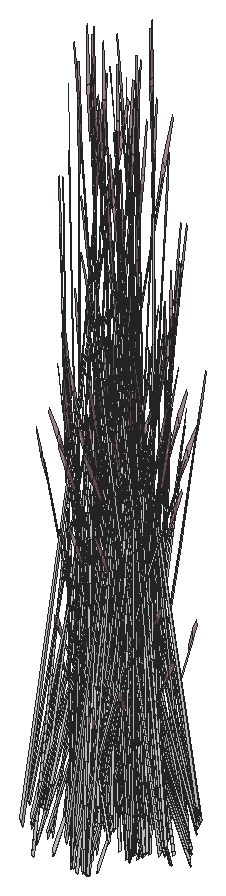
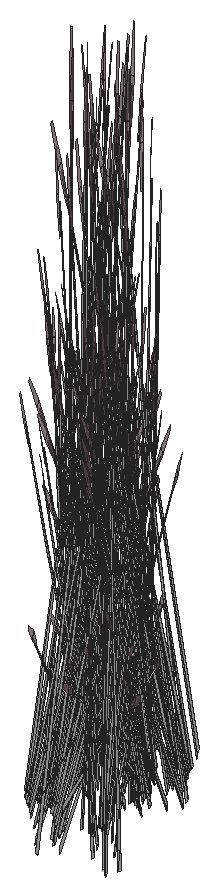
# SketchUp Ruby script. Lengths in inches.
U = 1.inch
M = Sketchup.active_model
def pt(a) = Geom::Point3d.new(a.map { |v| v * U })
def face(e, loops, mat)
  f = e.add_face(loops[0].map { |a| pt(a) })
  loops[1..].each { |l| e.add_face(l.map { |a| pt(a) }).erase! }
  f.material = f.back_material = mat if mat
  f
end
# faces: each face lists its corners as indices into pts; further lists are holes
def faces(e, pts, list, mat = nil) = list.each { |f| face(e, (f[0].is_a?(Array) ? f : [f]).map { |l| l.map { |i| pts[i] } }, mat) }
# xy, xz, yz: faces in a plane at the given z, y or x. An outline is a flat list of corners, or four numbers for a rectangle; further outlines are holes
def ring(l) = l.size == 4 ? [[l[0], l[1]], [l[2], l[1]], [l[2], l[3]], [l[0], l[3]]] : l.each_slice(2).to_a
def flat(e, list, mat, &to3) = list.each { |f| face(e, (f[0].is_a?(Array) ? f : [f]).map { |l| ring(l).map { |u, v| to3.(u, v) } }, mat) }
def xy(e, z, list, mat = nil) = flat(e, list, mat) { |x, y| [x, y, z] }
def xz(e, y, list, mat = nil) = flat(e, list, mat) { |x, z| [x, y, z] }
def yz(e, x, list, mat = nil) = flat(e, list, mat) { |y, z| [x, y, z] }
def lines(e, pts, list) = list.each { |a, b| e.add_line(pt(pts[a]), pt(pts[b])) }
# prism: a flat outline (further loops are holes) pulled along v
def prism(e, loops, v, mat = nil)
  f = face(e, loops, mat); d = Geom::Vector3d.new(v.map { |x| x * U })
  f.pushpull(f.normal.samedirection?(d) ? d.length : -d.length)
end
def box(e, o, s, mat = nil) = prism(e, [[o, [o[0] + s[0], o[1], o[2]], [o[0] + s[0], o[1] + s[1], o[2]], [o[0], o[1] + s[1], o[2]]]], [0, 0, s[2]], mat)
def at(x, y, z, deg = 0) = Geom::Transformation.translation(pt([x, y, z])) * Geom::Transformation.rotation(ORIGIN, Z_AXIS, deg.degrees)
def axes(o, x, y, z) = Geom::Transformation.new([*x, 0, *y, 0, *z, 0, *pt(o).to_a, 1])
def part(name) = M.definitions.add(name)
# library, detail: a bought-in or finely detailed component or shape, given as its bounding box
def library(name, o, s) = part(name).tap { |d| box(d.entities, o, s) }
def detail(e, o, s) = box(e.add_group.entities, o, s)
def put(e, d, t, mat = nil) = e.add_instance(d, t).tap { |i| i.material = mat if mat }
def group(e, t, mat = nil) = e.add_group.tap { |g| g.transformation = t; g.material = mat if mat }.entities
root = M.entities
M.materials.add("LightPink_Translucent").color = [144, 107, 117]
M.materials["LightPink_Translucent"].alpha = 0.75
c1 = part("blade")
p = [[2.15,0.21,22],[0,0.17,0],[0.09,0.45,0],[2.18,0.31,22],[2.29,0.31,22],[0.38,0.45,0],
  [2.48,0.24,33],[2.49,0.24,33],[2.48,0.22,33]]
faces(c1.entities,p,[[0,1,2,3],[4,5,2,3],[6,3,4,7],[8,0,3,6]])
c2 = part("seeds")
p = [[0.3,-0.1,1.38],[-0.01,-0.03,1.59],[-0.01,-0.03,0.03],[0.14,-0.07,-0.07],[0.29,-0.03,3],[0.15,0.01,3.11]]
faces(c2.entities,p,[[0,1,2,3],[1,0,4,5]],"LightPink_Translucent")
c3 = part("blade with seeds")
put(c3.entities,c1,at(0,0,0))
put(c3.entities,c2,axes([2.4,0.25,30.99],[1.5799,-0.05474,1.17369],[-0.12525,1.92788,0.29478],[-0.07173,-0.02425,1.56792]))
put(root,c3,axes([353.46,654.26,621.17],[-0.32928,-0.11539,-0.30978],[0.08291,-0.40636,0.30978],[-0.06638,0.04686,1.38974]))
put(root,c3,axes([350.63,652.3,623.57],[-0.1311,-0.08035,1.71376],[0.27131,-0.33708,0.13857],[0.16909,0.15206,0.73262]))
put(root,c3,axes([349.23,653.36,625.26],[0.21031,-0.39918,-0.1216],[0.30457,0.22997,-0.67495],[0.10587,0.11278,1.02557]))
put(root,c3,axes([355.72,653.76,623.51],[0.10032,-0.06746,1.77064],[0.0346,0.47103,0.13857],[-0.2173,0.0625,0.63284]))
put(root,c3,axes([350.66,651.24,624.16],[-0.30498,-0.24231,1.38283],[0.32203,-0.37727,0.59665],[0.0984,0.22736,1.33663]))
put(root,c3,axes([358.33,656.1875,622.9],[-0.36714,-0.07646,-0.62353],[0.07747,-0.47163,-0.16365],[-0.10956,-0.05715,1.37633]))
put(root,c3,axes([354.74,652.71,621.51],[0.44133,0,0],[0,0.52122,-0.51607],[0,0.11871,1.63711]))
put(root,c3,axes([354.56,652.97,621.34],[-0.44111,-0.00373,-0.04976],[0,-0.52122,0.49943],[-0.01386,0.11865,1.58352]))
put(root,c3,axes([353.61,652.52,621.8],[0.39748,0.22252,-0.29095],[-0.19139,0.46966,-0.50002],[0.01249,0.11531,1.59708]))
put(root,c3,axes([356.57,655.43,622.36],[-0.35581,-0.20937,0],[0.17124,-0.43505,0],[0,0,1.62707]))
put(root,c3,axes([356.86,654.87,622.63],[-0.34464,-0.37536,-0.25192],[0.29,-0.42149,0.5513],[-0.0928,0.04391,1.68216]))
put(root,c3,axes([355.95,655.59,622.65],[0.33032,0.23318,0.49651],[-0.19744,0.41812,0],[-0.07523,-0.05311,1.57504]))
put(root,c3,axes([351.12,653.22,622.46],[-0.19872,-0.13409,1.1486],[0.2566,-0.13625,0.84392],[0.06921,0.11541,0.25299]))
put(root,c3,axes([354.37,653.86,623.66],[0.20082,0.29199,-0.35414],[-0.2293,0.2764,0.4572],[0.1165,0.04206,0.87481]))
put(root,c3,axes([354.47,653.05,621.17],[-0.24637,0.29097,-0.30978],[-0.24637,-0.29097,0.30978],[0,0.09372,1.38974]))
put(root,c3,axes([350.42,653.6,624.73],[0.21031,-0.39918,-0.1216],[0.30457,0.22997,-0.67495],[0.10587,0.11278,1.02557]))
put(root,c3,axes([353.41,653.08,621.8],[0.04113,0.53214,-0.29095],[-0.42835,0.03218,-0.50002],[-0.07543,0.07088,1.59708]))
put(root,c3,axes([354.27,653.97,623.87],[-0.01777,0.35463,0.0643],[-0.26836,-0.00972,0.50621],[0.1028,0.03711,0.77189]))
put(root,c3,axes([357.18,655.31,625.58],[0.09971,-0.42522,0.48003],[0.32782,0.1454,0.3958],[-0.12892,0.02555,0.9933]))
put(root,c3,axes([353.5625,652.87,621.35],[-0.17124,0.42022,-0.44739],[-0.35581,-0.20224,0.21531],[0,0.09687,1.43643]))
put(root,c3,axes([349.98,653.48,621.72],[0.02571,-0.06733,1.76342],[0.32373,-0.19829,-0.26939],[0.09815,0.10263,0.30037]))
put(root,c3,axes([357.15,655.19,625.58],[-0.12963,-0.31798,0.0643],[0.23638,-0.15564,0.50621],[-0.1042,0.03071,0.77189]))
put(root,c3,axes([354.29,653.86,623.87],[-0.26024,0.30729,0.48003],[-0.22444,-0.32634,0.3958],[0.1221,0.05668,0.9933]))
put(root,c3,axes([349.48,653.16,624.91],[0.34827,-0.11086,-0.51099],[0.06092,0.41983,-0.3958],[0.09354,0.12031,0.97773]))
put(root,c3,axes([354.64,654.08,624.88],[-0.05763,0.06055,1.74944],[0.0049,0.44239,-0.27667],[-0.13211,0.05753,0.14031]))
put(root,c3,axes([355.03,654.02,624.85],[-0.09562,0.42421,-0.51099],[-0.32782,-0.1454,-0.3958],[-0.13199,0.0389,0.97773]))
put(root,c3,axes([355.01,653.66,625.2],[0.17758,0.42229,-0.1216],[-0.31518,0.20752,-0.67495],[-0.13282,0.05572,1.02557]))
put(root,c3,axes([357.15,655.52,622.34],[0.00895,0.0735,1.76342],[-0.18044,0.38382,-0.26939],[-0.12817,-0.01935,0.30037]))
put(root,c3,axes([355.76,655.83,622.54],[-0.22066,0.46731,0],[-0.36918,-0.26061,-0.51607],[-0.08408,-0.05936,1.63711]))
put(root,c3,axes([350.15,653.93,624.4],[0.00104,-0.05646,1.77383],[0.30246,-0.2491,-0.16761],[0.10506,0.08891,0.31391]))
put(root,c3,axes([351.18,653.71,621.18],[0.02571,-0.06733,1.76342],[0.32373,-0.19829,-0.26939],[0.09815,0.10263,0.30037]))
put(root,c3,axes([357.9375,656.9,622.875],[-0.08291,-0.40636,-0.30978],[0.32928,-0.11539,0.30978],[-0.06638,-0.04686,1.38974]))
put(root,c3,axes([350.75,652.18,621.79],[0.12941,0.42699,-0.69212],[-0.37279,0.15378,-0.18165],[0.0143,0.14459,1.52773]))
put(root,c3,axes([357.03,654.56,622.89],[0.38326,-0.02879,0.44739],[0.03466,0.47788,-0.21531],[-0.06861,0.04843,1.43643]))
put(root,c3,axes([349.96,653.59,622.89],[-0.22633,-0.01463,1.0506],[0.14947,-0.31064,0.58006],[0.08941,0.11036,0.8241]))
put(root,c3,axes([350.67,653.4,624.37],[0.34827,-0.11086,-0.51099],[0.06092,0.41983,-0.3958],[0.09354,0.12031,0.97773]))
put(root,c3,axes([353.15,653.48,621.2],[-0.23773,0.35053,-0.62353],[-0.29532,-0.31785,-0.16365],[-0.09526,0.08744,1.37633]))
put(root,c3,axes([353.47,654.22,624.1875],[-0.05451,-0.37564,0.35414],[0.31161,-0.09919,-0.4572],[0.0837,0.10765,0.87481]))
put(root,c3,axes([356.6875,654.79,622.38],[-0.38326,0.02879,-0.44739],[-0.03466,-0.47788,0.21531],[-0.06861,0.04843,1.43643]))
put(root,c3,axes([353.57,654.08,621.47],[0.44186,0.15158,0.30756],[-0.11054,0.54181,-0.36492],[-0.07313,0.06781,1.64885]))
put(root,c3,axes([353.54,654.44,621.16],[-0.33032,0.23318,-0.49651],[-0.19744,-0.41812,0],[-0.07523,0.05311,1.57504]))
put(root,c3,axes([354.64,653.0625,621.16],[0,0.46636,-0.49651],[-0.39487,0,0],[0,0.10622,1.57504]))
put(root,c3,axes([353.65,653.11,623.01],[-0.1311,-0.08035,1.71376],[0.27131,-0.33708,0.13857],[0.16909,0.15206,0.73262]))
put(root,c3,axes([357.85,657.08,622.86],[-0.33032,-0.23318,-0.49651],[0.19744,-0.41812,0],[-0.07523,-0.05311,1.57504]))
put(root,c3,axes([357.11,655.35,625.37],[-0.29332,-0.1301,-0.35414],[0.08555,-0.37955,0.4572],[-0.11809,0.0348,0.87481]))
put(root,c3,axes([351.15,653.83,622.36],[-0.22633,-0.01463,1.0506],[0.14947,-0.31064,0.58006],[0.08941,0.11036,0.8241]))
put(root,c3,axes([353.68,652.06,623.61],[-0.30498,-0.24231,1.38283],[0.32203,-0.37727,0.59665],[0.0984,0.22736,1.33663]))
put(root,c3,axes([358.74,656.26,623.51],[-0.35635,0.30962,-0.29095],[-0.23697,-0.43749,-0.50002],[-0.08792,-0.04443,1.59708]))
put(root,c3,axes([350.5,653.74,624.42],[-0.16041,0.29625,0.0643],[-0.22843,-0.17248,0.50621],[0.07385,0.09498,0.77189]))
put(root,c3,axes([354.14,654.03,621.9],[-0.19872,-0.13409,1.1486],[0.2566,-0.13625,0.84392],[0.06921,0.11541,0.25299]))
put(root,c3,axes([353.4375,654.41,624.17],[0.21031,-0.39918,-0.1216],[0.30457,0.22997,-0.67495],[0.10587,0.11278,1.02557]))
put(root,c3,axes([350.57,653.66,624.42],[-0.35104,0.10702,0.48003],[-0.06092,-0.41983,0.3958],[0.08256,0.12373,0.9933]))
put(root,c3,axes([357.11,655.9,622.36],[-0.21791,-0.46895,-0.05142],[0.36918,-0.26061,0.51607],[-0.09097,0.04465,1.6363]))
put(root,c3,axes([357.03,654.77,622.79],[0.26075,0.2802,0.1448],[-0.2175,0.31612,-0.41347],[-0.06054,0.04274,1.26744]))
put(root,c3,axes([354.97,654.84,624.9],[-0.08753,-0.42921,0.48003],[0.34336,-0.07449,0.3958],[-0.1012,0.10094,0.9933]))
put(root,c3,axes([354.91,654.76,624.9],[-0.2423,-0.19613,0.0643],[0.14107,-0.2793,0.50621],[-0.07768,0.0903,0.77189]))
put(root,c3,axes([355.02,654.24,624.04],[0.12246,-0.09864,1.71376],[0.1031,0.45582,0.13857],[-0.19225,0.10302,0.73262]))
put(root,c3,axes([352.05,653.87,624.1875],[0.23881,-0.24554,0.35414],[0.22606,0.28036,-0.4572],[-0.0344,0.14245,0.87481]))
put(root,c3,axes([350.41,653.07,622.28],[0.00623,-0.15459,1.43002],[0.29764,-0.17268,-0.30754],[0.09188,0.18503,0.61141]))
put(root,c3,axes([353.84,654.37,621.51],[0.22066,0.46731,0],[-0.36918,0.26061,-0.51607],[-0.08408,0.05936,1.63711]))
put(root,c3,axes([357.42,655.3125,625.9],[0.29332,0.1301,0.35414],[-0.08555,0.37955,-0.4572],[-0.11809,0.0348,0.87481]))
put(root,c3,axes([353.16,654.74,623.85],[0.00104,-0.05646,1.77383],[0.30246,-0.2491,-0.16761],[0.10506,0.08891,0.31391]))
put(root,c3,axes([354.19,654.53,620.63],[0.02571,-0.06733,1.76342],[0.32373,-0.19829,-0.26939],[0.09815,0.10263,0.30037]))
put(root,c3,axes([353.65,652.52,621.98],[-0.00964,-0.43909,1.41272],[0.43635,0.11382,0.59816],[-0.1032,0.24027,1.3335]))
put(root,c3,axes([353.76,653,621.23],[0.12941,0.42699,-0.69212],[-0.37279,0.15378,-0.18165],[0.0143,0.14459,1.52773]))
put(root,c3,axes([353.6875,654.21,623.82],[0.34827,-0.11086,-0.51099],[0.06092,0.41983,-0.3958],[0.09354,0.12031,0.97773]))
put(root,c3,axes([357.3125,655.63,622.65],[0.33032,-0.23318,0.49651],[0.19744,0.41812,0],[-0.07523,0.05311,1.57504]))
put(root,c3,axes([352.72,654.28,624.1875],[0.1064,-0.35863,0.35414],[0.31043,0.1046,-0.4572],[0.02846,0.14439,0.87481]))
put(root,c3,axes([358,655.29,624.1875],[0.10032,-0.06746,1.77064],[0.0346,0.47103,0.13857],[-0.2173,0.0625,0.63284]))
put(root,c3,axes([357.01,655.84,622.2],[-0.32928,-0.11539,-0.30978],[0.08291,-0.40636,0.30978],[-0.06638,0.04686,1.38974]))
put(root,c3,axes([354.64,655.02,622.76],[0.12266,0.03828,1.43002],[0.07906,0.39104,-0.30754],[-0.16661,0.0732,0.61141]))
put(root,c3,axes([350.82,660.1,620.59],[-0.10032,0.0944,1.43002],[-0.30046,-0.16522,-0.30754],[0.05569,-0.20547,0.61141]))
put(root,c3,axes([355.1875,654.7,625.22],[0.30722,-0.06665,0.35414],[0.08112,0.381,-0.4572],[-0.08804,0.10234,0.87481]))
put(root,c3,axes([354.17,654.64,621.8],[-0.22633,-0.01463,1.0506],[0.14947,-0.31064,0.58006],[0.08941,0.11036,0.8241]))
put(root,c3,axes([354,654.53,624.88],[0.04504,0.01251,1.77383],[0.13934,0.41205,-0.16761],[-0.0922,0.10815,0.31391]))
put(root,c3,axes([355.53,660.61,621.875],[0.08068,0.14973,1.71376],[-0.3728,0.12606,0.13857],[-0.08426,-0.23506,0.73262]))
put(root,c3,axes([357.66,660.63,621.875],[0.08068,0.14973,1.71376],[-0.3728,0.12606,0.13857],[-0.08426,-0.23506,0.73262]))
put(root,c3,axes([353.52,654.56,623.87],[-0.16041,0.29625,0.0643],[-0.22843,-0.17248,0.50621],[0.07385,0.09498,0.77189]))
put(root,c3,axes([354.38,655.84,622.93],[0.14709,-0.21136,1.1486],[0.05804,0.3346,0.84392],[-0.1063,0.05991,0.25299]))
put(root,c3,axes([356.15,659.62,622.72],[-0.05398,-0.06539,1.74944],[-0.36026,0.04145,-0.27667],[-0.0575,-0.15639,0.14031]))
put(root,c3,axes([356.96,654.66,622.83],[0.04113,0.53214,-0.29095],[-0.42835,0.03218,-0.50002],[-0.07543,0.07088,1.59708]))
put(root,c3,axes([353.14,655.55,624.78],[0.2439,-0.26754,-0.06488],[0.22348,0.29302,-0.29416],[0.01573,0.08303,0.97024]))
put(root,c3,axes([357.11,654.45,622.38],[-0.17124,0.42022,-0.44739],[-0.35581,-0.20224,0.21531],[0,0.09687,1.43643]))
put(root,c3,axes([350.09,652.77,623.57],[-0.08068,-0.14973,1.71376],[0.3728,-0.12606,0.13857],[0.08426,0.23506,0.73262]))
put(root,c3,axes([353.58,654.47,623.87],[-0.35104,0.10702,0.48003],[-0.06092,-0.41983,0.3958],[0.08256,0.12373,0.9933]))
put(root,c3,axes([354.93,654.92,624.7],[-0.30722,0.06665,-0.35414],[-0.08112,-0.381,0.4572],[-0.08804,0.10234,0.87481]))
put(root,c3,axes([356.53,660.73,622.98],[-0.16845,-0.3792,-0.71045],[0.34676,-0.21133,0.08574],[-0.03939,-0.18322,1.00501]))
put(root,c3,axes([356.93,655.61,625.56],[-0.05763,0.06055,1.74944],[0.0049,0.44239,-0.27667],[-0.13211,0.05753,0.14031]))
put(root,c3,axes([357.3125,655.55,625.53],[-0.09562,0.42421,-0.51099],[-0.32782,-0.1454,-0.3958],[-0.13199,0.0389,0.97773]))
put(root,c3,axes([357.3,655.18,625.88],[0.17758,0.42229,-0.1216],[-0.31518,0.20752,-0.67495],[-0.13282,0.05572,1.02557]))
put(root,c3,axes([351.06,660.8,622.98],[0.00918,-0.43138,-0.71045],[0.38672,0.02897,0.08574],[0.04081,-0.18275,1.00501]))
put(root,c3,axes([355.43,660.22,620.59],[-0.02137,0.15256,1.43002],[-0.31245,0.12771,-0.30754],[-0.07303,-0.19719,0.61141]))
put(root,c3,axes([358.05,657.36,623.22],[-0.22066,0.46731,0],[-0.36918,-0.26061,-0.51607],[-0.08408,-0.05936,1.63711]))
put(root,c3,axes([357.56,660.23,620.59],[-0.02137,0.15256,1.43002],[-0.31245,0.12771,-0.30754],[-0.07303,-0.19719,0.61141]))
put(root,c3,axes([353.43,653.88,621.73],[0.00623,-0.15459,1.43002],[0.29764,-0.17268,-0.30754],[0.09188,0.18503,0.61141]))
put(root,c3,axes([351.6,660.12,622.72],[-0.00341,-0.09282,1.74944],[-0.28775,-0.26825,-0.27667],[0.04449,-0.16261,0.14031]))
put(root,c3,axes([350.625,660.58,621.875],[-0.06572,0.16029,1.71376],[-0.27569,-0.33172,0.13857],[0.12437,-0.20675,0.73262]))
put(root,c3,axes([351.52,659.79,622.71],[-0.03584,0.03562,1.77383],[-0.35118,-0.12018,-0.16761],[-0.01271,-0.15545,0.31391]))
put(root,c3,axes([356.23,659.88,619.49],[-0.0592,0.0168,1.76342],[-0.32738,-0.18913,-0.26939],[0.00549,-0.15776,0.30037]))
put(root,c3,axes([352.625,654.6,623.87],[-0.26007,0.1585,0.0643],[-0.12729,-0.28902,0.50621],[0.02512,0.1274,0.77189]))
put(root,c3,axes([354.49,655.78,625.81],[0.31145,0.12449,-0.06488],[-0.0958,0.38314,-0.29416],[-0.05094,0.05817,0.97024]))
put(root,c3,axes([356.7,655.07,622.23],[-0.23773,0.35053,-0.62353],[-0.29532,-0.31785,-0.16365],[-0.09526,0.08744,1.37633]))
put(root,c3,axes([351.9,653.9375,624.53],[0.3879,0.02311,-0.13498],[-0.0106,0.43749,-0.74919],[-0.02694,0.1685,1.13838]))
put(root,c3,axes([352.62,654.43,624.17],[0.34538,-0.21713,-0.1216],[0.16972,0.38536,-0.67495],[0.04557,0.16239,1.02557]))
put(root,c3,axes([352.72,654.57,624.2],[-0.34777,-0.12192,0.53283],[0.11892,-0.40083,0.43934],[0.0209,0.15763,1.10256]))
put(root,c3,axes([352.08,655.17,621.9],[-0.00913,-0.2773,1.1486],[0.22824,0.19778,0.84392],[-0.04489,0.13217,0.25299]))
put(root,c3,axes([357.12,655.66,622.5],[0.44186,0.15158,0.30756],[-0.11054,0.54181,-0.36492],[-0.07313,0.06781,1.64885]))
put(root,c3,axes([357.09,656.02,622.1875],[-0.33032,0.23318,-0.49651],[-0.19744,-0.41812,0],[-0.07523,0.05311,1.57504]))
put(root,c3,axes([350.98,660.65,622.68],[-0.25266,-0.31335,-0.51099],[0.2669,-0.27442,-0.3958],[0.03844,-0.15921,0.97773]))
put(root,c3,axes([356.56,660.4,622.53],[0.1064,-0.35863,-0.35414],[0.31043,0.1046,0.4572],[-0.02846,-0.14439,0.87481]))
put(root,c3,axes([352.68,654.51,620.63],[0.05712,-0.02538,1.76342],[0.34359,0.13968,-0.26939],[0.01005,0.15742,0.30037]))
put(root,c3,axes([355.03,654.66,625.2],[0.32648,0.25715,-0.1216],[-0.18809,0.3724,-0.67495],[-0.09224,0.12945,1.02557]))
put(root,c3,axes([356.4,660.65,622.68],[-0.34695,-0.11691,-0.51099],[0.11892,-0.40083,-0.3958],[-0.03181,-0.16138,0.97773]))
put(root,c3,axes([352.16,654.1,624.14],[0.25266,0.31335,-0.5672],[-0.2669,0.27442,-0.43934],[-0.03844,0.15921,1.08528]))
put(root,c3,axes([357.26,656.36,625.58],[-0.08753,-0.42921,0.48003],[0.34336,-0.07449,0.3958],[-0.1012,0.10094,0.9933]))
put(root,c3,axes([351.89,654.57,621.96],[0.32063,-0.08258,0.06507],[0.07371,0.33271,-0.86304],[-0.02033,0.16842,0.7736]))
put(root,c3,axes([357.19,656.28,625.58],[-0.2423,-0.19613,0.0643],[0.14107,-0.2793,0.50621],[-0.07768,0.0903,0.77189]))
put(root,c3,axes([352.91,654.41,623.82],[0.34695,0.11691,-0.51099],[-0.11892,0.40083,-0.3958],[0.03181,0.16138,0.97773]))
put(root,c3,axes([357.3,655.77,624.72],[0.12246,-0.09864,1.71376],[0.1031,0.45582,0.13857],[-0.19225,0.10302,0.73262]))
put(root,c3,axes([353.11,653.58,623.01],[-0.08068,-0.14973,1.71376],[0.3728,-0.12606,0.13857],[0.08426,0.23506,0.73262]))
put(root,c3,axes([355.47,654.55,624.04],[0.08815,-0.14329,1.71376],[0.22258,0.38678,0.13857],[-0.15267,0.17614,0.73262]))
put(root,c3,axes([351.25,660.82,623.03],[-0.3879,-0.02311,-0.1216],[0.0106,-0.43749,-0.67495],[0.02694,-0.1685,1.02557]))
put(root,c3,axes([355.78,659.41,622.71],[-0.00658,0.0559,1.77383],[-0.32474,0.20287,-0.16761],[-0.09556,-0.1037,0.31391]))
put(root,c3,axes([351.22,660.54,622.53],[0.23881,-0.24554,-0.35414],[0.22606,0.28036,0.4572],[0.0344,-0.14245,0.87481]))
put(root,c3,axes([355.1875,654.97,624.85],[0.09067,0.42583,-0.51099],[-0.34336,0.07449,-0.3958],[-0.0984,0.11438,0.97773]))
put(root,c3,axes([357.91,659.42,622.71],[-0.00658,0.0559,1.77383],[-0.32474,0.20287,-0.16761],[-0.09556,-0.1037,0.31391]))
put(root,c3,axes([355.6,655.46,625.22],[0.23881,-0.24554,0.35414],[0.22606,0.28036,-0.4572],[-0.0344,0.14245,0.87481]))
put(root,c3,axes([357.39,655.95,622.54],[0.22066,0.46731,0],[-0.36918,0.26061,-0.51607],[-0.08408,0.05936,1.63711]))
put(root,c3,axes([352.76,654.65,623.66],[-0.1064,0.35863,-0.35414],[-0.31043,-0.1046,0.4572],[0.02846,0.14439,0.87481]))
put(root,c3,axes([355.71,660.4,623.09],[0.39316,-0.11987,0.53763],[0.06823,0.47021,0.4433],[-0.09247,-0.13858,1.11249]))
put(root,c3,axes([357.83,660.41,623.09],[0.39316,-0.11987,0.53763],[0.06823,0.47021,0.4433],[-0.09247,-0.13858,1.11249]))
put(root,c3,axes([357.2,654.1,623.01],[-0.00964,-0.43909,1.41272],[0.43635,0.11382,0.59816],[-0.1032,0.24027,1.3335]))
put(root,c3,axes([355.38,655.68,624.9],[-0.29004,-0.02173,0.0643],[0.00795,-0.32812,0.50621],[-0.03035,0.12569,0.77189]))
put(root,c3,axes([354.77,656.05,621.66],[0.04734,0.04659,1.76342],[0.08027,0.4317,-0.26939],[-0.10492,0.09206,0.30037]))
put(root,c3,axes([352.09,653.96,624.48],[-0.00918,0.43138,-0.7886],[-0.38672,-0.02897,0.09517],[-0.04081,0.18275,1.11556]))
put(root,c3,axes([356.6,660.49,622.73],[0.34777,0.12192,0.48003],[-0.11892,0.40083,0.3958],[-0.0209,-0.15763,0.9933]))
put(root,c3,axes([355.48,655.71,624.9],[-0.25132,-0.3182,0.48003],[0.2669,-0.27442,0.3958],[-0.04636,0.14929,0.9933]))
put(root,c3,axes([351.08,655.09,623.85],[0.04004,-0.02816,1.77383],[0.33095,0.18728,-0.16761],[-0.00778,0.15594,0.31391]))
put(root,c3,axes([356.7,660.63,623.03],[-0.34538,0.21713,-0.1216],[-0.16972,-0.38536,-0.67495],[-0.04557,-0.16239,1.02557]))
put(root,c3,axes([355.32,659.97,620.77],[0.18411,0.16231,1.1486],[-0.26813,0.09757,0.84392],[-0.05737,-0.12474,0.25299]))
put(root,c3,axes([356.6875,660.46,622.73],[0.26007,-0.1585,0.0643],[0.12729,0.28902,0.50621],[-0.02512,-0.1274,0.77189]))
put(root,c3,axes([357.45,659.99,620.77],[0.18411,0.16231,1.1486],[-0.26813,0.09757,0.84392],[-0.05737,-0.12474,0.25299]))
put(root,c3,axes([355.77,660.83,622.98],[-0.30095,-0.22541,-0.71045],[0.21388,-0.395,0.08574],[-0.10904,-0.13459,1.00501]))
put(root,c3,axes([356.92,656.54,623.4375],[0.12266,0.03828,1.43002],[0.07906,0.39104,-0.30754],[-0.16661,0.0732,0.61141]))
put(root,c3,axes([357.89,660.85,622.98],[-0.30095,-0.22541,-0.71045],[0.21388,-0.395,0.08574],[-0.10904,-0.13459,1.00501]))
put(root,c3,axes([355.66,660.54,622.53],[-0.05451,-0.37564,-0.35414],[0.31161,-0.09919,0.4572],[-0.0837,-0.10765,0.87481]))
put(root,c3,axes([357.79,660.55,622.53],[-0.05451,-0.37564,-0.35414],[0.31161,-0.09919,0.4572],[-0.0837,-0.10765,0.87481]))
put(root,c3,axes([352.45,653.65,623.01],[-0.00864,-0.17899,1.71376],[0.37441,0.11874,0.13857],[-0.02316,0.25508,0.73262]))
put(root,c3,axes([357.47,656.22,625.9],[0.30722,-0.06665,0.35414],[0.08112,0.381,-0.4572],[-0.08804,0.10234,0.87481]))
put(root,c3,axes([356.29,656.05,625.55],[0.04504,0.01251,1.77383],[0.13934,0.41205,-0.16761],[-0.0922,0.10815,0.31391]))
put(root,c3,axes([356.66,657.36,623.61],[0.14709,-0.21136,1.1486],[0.05804,0.3346,0.84392],[-0.1063,0.05991,0.25299]))
put(root,c3,axes([351.52,660.39,619.49],[-0.05283,-0.03674,1.76342],[-0.13569,-0.41045,-0.26939],[0.09154,-0.11138,0.30037]))
put(root,c3,axes([352.79,654.33,624.12],[0.16845,0.3792,-0.71045],[-0.34676,0.21133,0.08574],[0.03939,0.18322,1.00501]))
put(root,c3,axes([357.22,656.45,625.37],[-0.30722,0.06665,-0.35414],[-0.08112,-0.381,0.4572],[-0.08804,0.10234,0.87481]))
put(root,c3,axes([355.8,660.5,622.73],[0.16041,-0.29625,0.0643],[0.22843,0.17248,0.50621],[-0.07385,-0.09498,0.77189]))
put(root,c3,axes([355.18,660.46,619.49],[-0.03419,0.06144,1.76342],[-0.3455,0.13246,-0.26939],[-0.08346,-0.12049,0.30037]))
put(root,c3,axes([352.54,655.29,623.85],[0.04474,0.0751,1.74944],[0.36104,0.0295,-0.27667],[0.03631,0.16562,0.14031]))
put(root,c3,axes([357.3,660.48,619.49],[-0.03419,0.06144,1.76342],[-0.3455,0.13246,-0.26939],[-0.08346,-0.12049,0.30037]))
put(root,c3,axes([351.22,660.63,622.73],[0.25132,0.3182,0.48003],[-0.2669,0.27442,0.3958],[0.04636,-0.14929,0.9933]))
put(root,c3,axes([355.4,654.9,624.04],[0.06572,-0.16029,1.71376],[0.27569,0.33172,0.13857],[-0.12437,0.20675,0.73262]))
put(root,c3,axes([351.3125,660.66,622.73],[0.29004,0.02173,0.0643],[-0.00795,0.32812,0.50621],[0.03035,-0.12569,0.77189]))
put(root,c3,axes([355.75,662.15,620.1],[-0.14494,-0.47823,-0.69835],[0.41752,-0.17223,-0.18329],[-0.01602,-0.16194,1.54149]))
put(root,c3,axes([354.99,661.08,621.875],[0.1311,0.08035,1.71376],[-0.27131,0.33708,0.13857],[-0.16909,-0.15206,0.73262]))
put(root,c3,axes([357.12,661.1,621.875],[0.1311,0.08035,1.71376],[-0.27131,0.33708,0.13857],[-0.16909,-0.15206,0.73262]))
put(root,c3,axes([351.09,660.89,623.05],[-0.23881,0.24554,0.35414],[-0.22606,-0.28036,-0.4572],[0.0344,-0.14245,0.87481]))
put(root,c3,axes([356.77,657.3,626.49],[0.31145,0.12449,-0.06488],[-0.0958,0.38314,-0.29416],[-0.05094,0.05817,0.97024]))
put(root,c3,axes([351.52,661.55,622.98],[0.18436,-0.36797,-0.71045],[0.32306,0.26151,0.08574],[0.11008,-0.13332,1.00501]))
put(root,c3,axes([356.17,656.18,624.9],[-0.26007,0.1585,0.0643],[-0.12729,-0.28902,0.50621],[0.02512,0.1274,0.77189]))
put(root,c3,axes([356.59,660.78,623.05],[-0.1064,0.35863,0.35414],[-0.31043,-0.1046,-0.4572],[-0.02846,-0.14439,0.87481]))
put(root,c3,axes([351.51,661.375,622.68],[-0.09067,-0.42583,-0.51099],[0.34336,-0.07449,-0.3958],[0.0984,-0.11438,0.97773]))
put(root,c3,axes([355.48,655.8,624.7],[-0.23881,0.24554,-0.35414],[-0.22606,-0.28036,0.4572],[-0.0344,0.14245,0.87481]))
put(root,c3,axes([354.65,655.73,624.88],[-0.00877,0.09229,1.74944],[0.24897,0.32105,-0.27667],[-0.06518,0.15182,0.14031]))
put(root,c3,axes([355.45,655.52,625.57],[0.3879,0.02311,-0.13498],[-0.0106,0.43749,-0.74919],[-0.02694,0.1685,1.13838]))
put(root,c3,axes([355.625,660.84,622.68],[-0.34827,0.11086,-0.51099],[-0.06092,-0.41983,-0.3958],[-0.09354,-0.12031,0.97773]))
put(root,c3,axes([356.27,656.15,625.23],[-0.34777,-0.12192,0.53283],[0.11892,-0.40083,0.43934],[0.0209,0.15763,1.10256]))
put(root,c3,axes([357.75,660.86,622.68],[-0.34827,0.11086,-0.51099],[-0.06092,-0.41983,-0.3958],[-0.09354,-0.12031,0.97773]))
put(root,c3,axes([355.87,660.47,623.43],[-0.23555,0.44708,-0.13619],[-0.34112,-0.25757,-0.75594],[-0.11858,-0.12631,1.14864]))
put(root,c3,axes([358,660.49,623.43],[-0.23555,0.44708,-0.13619],[-0.34112,-0.25757,-0.75594],[-0.11858,-0.12631,1.14864]))
put(root,c3,axes([355.63,656.76,622.93],[-0.00913,-0.2773,1.1486],[0.22824,0.19778,0.84392],[-0.04489,0.13217,0.25299]))
put(root,c3,axes([351.67,661.68,623.03],[-0.32648,-0.25715,-0.1216],[0.18809,-0.3724,-0.67495],[0.09224,-0.12945,1.02557]))
put(root,c3,axes([351.96,654.57,622.5],[0.00775,-0.24075,1.54345],[0.34877,0.12716,0.21329],[-0.03022,0.25658,0.72882]))
put(root,c3,axes([356.23,656.09,621.66],[0.05712,-0.02538,1.76342],[0.34359,0.13968,-0.26939],[0.01005,0.15742,0.30037]))
put(root,c3,axes([357.31,656.1875,625.88],[0.32648,0.25715,-0.1216],[-0.18809,0.3724,-0.67495],[-0.09224,0.12945,1.02557]))
put(root,c3,axes([356.17,660.21,620.13],[-0.2439,0.26754,-0.03893],[-0.22348,-0.29302,-0.17649],[-0.01573,-0.08303,0.58215]))
put(root,c3,axes([355.71,655.6875,625.17],[0.25266,0.31335,-0.5672],[-0.2669,0.27442,-0.43934],[-0.03844,0.15921,1.08528]))
put(root,c3,axes([357.75,656.07,624.72],[0.08815,-0.14329,1.71376],[0.22258,0.38678,0.13857],[-0.15267,0.17614,0.73262]))
put(root,c3,axes([355.4375,656.16,622.99],[0.32063,-0.08258,0.06507],[0.07371,0.33271,-0.86304],[-0.02033,0.16842,0.7736]))
put(root,c3,axes([354.97,660.34,622.72],[-0.07594,-0.00329,1.74944],[-0.24177,0.32918,-0.27667],[-0.129,-0.06726,0.14031]))
put(root,c3,axes([349.82,660.4,620.02],[0.33032,-0.23318,-0.49651],[0.19744,0.41812,0],[0.07523,-0.05311,1.57504]))
put(root,c3,axes([357.47,656.49,625.53],[0.09067,0.42583,-0.51099],[-0.34336,0.07449,-0.3958],[-0.0984,0.11438,0.97773]))
put(root,c3,axes([357.09,660.36,622.72],[-0.07594,-0.00329,1.74944],[-0.24177,0.32918,-0.27667],[-0.129,-0.06726,0.14031]))
put(root,c3,axes([351.78,661.21,620.59],[-0.12609,-0.01381,1.43002],[-0.12917,-0.37055,-0.30754],[0.1549,-0.10482,0.61141]))
put(root,c3,axes([352.47,661.57,622.71],[-0.0461,-0.00354,1.77383],[-0.19143,-0.37951,-0.16761],[0.07688,-0.12478,0.31391]))
put(root,c3,axes([350.21,661.36,620.06],[0.23773,-0.35053,-0.62353],[0.29532,0.31785,-0.16365],[0.09526,-0.08744,1.37633]))
put(root,c3,axes([356.3,656.24,624.7],[-0.1064,0.35863,-0.35414],[-0.31043,-0.1046,0.4572],[0.02846,0.14439,0.87481]))
put(root,c3,axes([351.93,660.53,620.77],[-0.11756,0.2374,1.1486],[-0.10105,-0.31895,0.84392],[0.09709,-0.07992,0.25299]))
